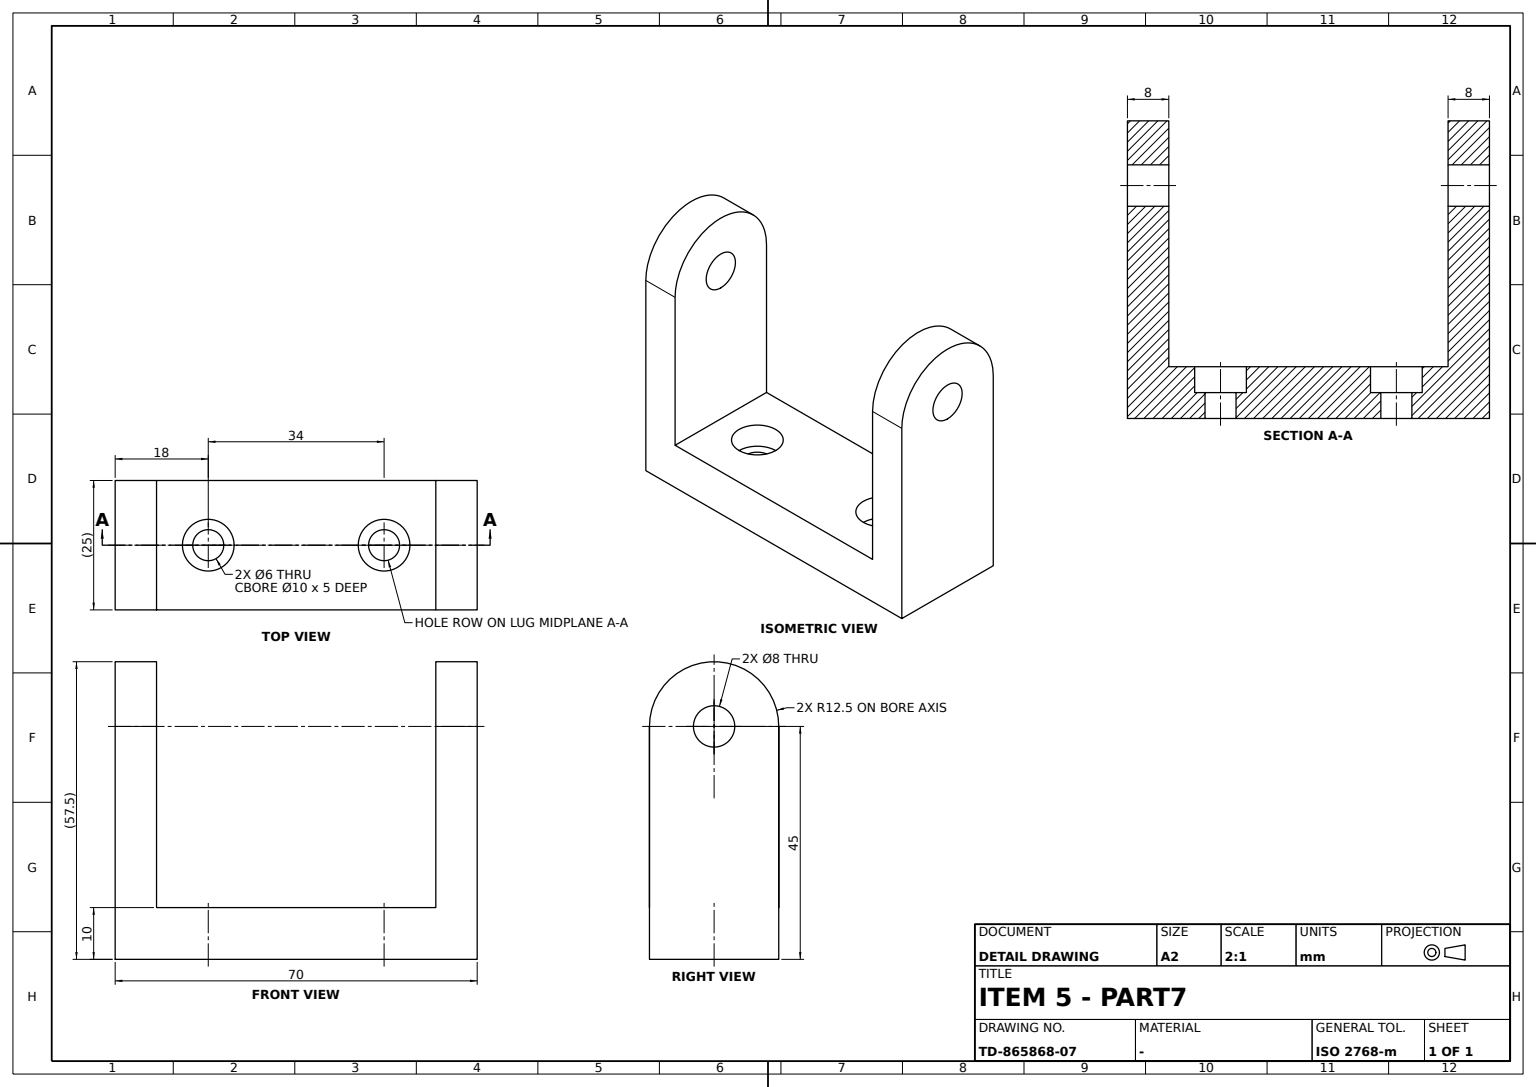
ISO-10303-21;
HEADER;
FILE_DESCRIPTION((''),'2;1');
FILE_NAME('','',(''),(''),'','','');
FILE_SCHEMA(('AUTOMOTIVE_DESIGN'));
ENDSEC;
DATA;
#1=APPLICATION_CONTEXT('');
#2=PRODUCT_CONTEXT('',#1,'mechanical');
#3=PRODUCT('','','',(#2));
#4=PRODUCT_DEFINITION_FORMATION('','',#3);
#5=PRODUCT_DEFINITION_CONTEXT('',#1,'design');
#6=PRODUCT_DEFINITION('','',#4,#5);
#7=PRODUCT_DEFINITION_SHAPE('','',#6);
#8=(LENGTH_UNIT()NAMED_UNIT(*)SI_UNIT(.MILLI.,.METRE.));
#9=(NAMED_UNIT(*)PLANE_ANGLE_UNIT()SI_UNIT($,.RADIAN.));
#10=(NAMED_UNIT(*)SI_UNIT($,.STERADIAN.)SOLID_ANGLE_UNIT());
#11=UNCERTAINTY_MEASURE_WITH_UNIT(LENGTH_MEASURE(0.005),#8,'distance_accuracy_value','');
#12=(GEOMETRIC_REPRESENTATION_CONTEXT(3)GLOBAL_UNCERTAINTY_ASSIGNED_CONTEXT((#11))GLOBAL_UNIT_ASSIGNED_CONTEXT((#8,#9,#10))REPRESENTATION_CONTEXT('',''));
#13=CARTESIAN_POINT('',(35.,0.,41.));
#14=VERTEX_POINT('',#13);
#15=CARTESIAN_POINT('',(35.,0.,45.));
#16=DIRECTION('',(1.,0.,0.));
#17=DIRECTION('',(0.,0.,-1.));
#18=AXIS2_PLACEMENT_3D('',#15,#16,#17);
#19=CIRCLE('',#18,4.);
#20=EDGE_CURVE('',#14,#14,#19,.T.);
#21=ORIENTED_EDGE('',*,*,#20,.F.);
#22=EDGE_LOOP('',(#21));
#23=FACE_BOUND('',#22,.T.);
#24=CARTESIAN_POINT('',(35.,12.5,0.));
#25=VERTEX_POINT('',#24);
#26=CARTESIAN_POINT('',(35.,12.5,45.));
#27=VERTEX_POINT('',#26);
#28=DIRECTION('',(0.,0.,1.));
#29=VECTOR('',#28,1000.);
#30=LINE('',#24,#29);
#31=EDGE_CURVE('',#25,#27,#30,.T.);
#32=ORIENTED_EDGE('',*,*,#31,.T.);
#33=CARTESIAN_POINT('',(35.,-12.5,45.));
#34=VERTEX_POINT('',#33);
#35=CIRCLE('',#18,12.5);
#36=EDGE_CURVE('',#27,#34,#35,.T.);
#37=ORIENTED_EDGE('',*,*,#36,.T.);
#38=CARTESIAN_POINT('',(35.,-12.5,0.));
#39=VERTEX_POINT('',#38);
#40=VECTOR('',#17,1000.);
#41=LINE('',#38,#40);
#42=EDGE_CURVE('',#34,#39,#41,.T.);
#43=ORIENTED_EDGE('',*,*,#42,.T.);
#44=CARTESIAN_POINT('',(35.,0.,0.));
#45=DIRECTION('',(0.,1.,0.));
#46=VECTOR('',#45,1000.);
#47=LINE('',#44,#46);
#48=EDGE_CURVE('',#39,#25,#47,.T.);
#49=ORIENTED_EDGE('',*,*,#48,.T.);
#50=EDGE_LOOP('',(#32,#37,#43,#49));
#51=FACE_BOUND('',#50,.T.);
#52=AXIS2_PLACEMENT_3D('',#44,#16,#45);
#53=PLANE('',#52);
#54=ADVANCED_FACE('',(#23,#51),#53,.T.);
#55=CARTESIAN_POINT('',(-27.,12.5,45.));
#56=VERTEX_POINT('',#55);
#57=CARTESIAN_POINT('',(-27.,-12.5,45.));
#58=VERTEX_POINT('',#57);
#59=CARTESIAN_POINT('',(-27.,0.,45.));
#60=AXIS2_PLACEMENT_3D('',#59,#16,#17);
#61=CIRCLE('',#60,12.5);
#62=EDGE_CURVE('',#56,#58,#61,.T.);
#63=ORIENTED_EDGE('',*,*,#62,.F.);
#64=CARTESIAN_POINT('',(-35.,12.5,45.));
#65=VERTEX_POINT('',#64);
#66=CARTESIAN_POINT('',(0.,12.5,45.));
#67=VECTOR('',#16,1000.);
#68=LINE('',#66,#67);
#69=EDGE_CURVE('',#65,#56,#68,.T.);
#70=ORIENTED_EDGE('',*,*,#69,.F.);
#71=CARTESIAN_POINT('',(-35.,-12.5,45.));
#72=VERTEX_POINT('',#71);
#73=CARTESIAN_POINT('',(-35.,0.,45.));
#74=AXIS2_PLACEMENT_3D('',#73,#16,#17);
#75=CIRCLE('',#74,12.5);
#76=EDGE_CURVE('',#65,#72,#75,.T.);
#77=ORIENTED_EDGE('',*,*,#76,.T.);
#78=CARTESIAN_POINT('',(0.,-12.5,45.));
#79=LINE('',#78,#67);
#80=EDGE_CURVE('',#72,#58,#79,.T.);
#81=ORIENTED_EDGE('',*,*,#80,.T.);
#82=EDGE_LOOP('',(#63,#70,#77,#81));
#83=FACE_BOUND('',#82,.T.);
#84=CARTESIAN_POINT('',(0.,0.,45.));
#85=AXIS2_PLACEMENT_3D('',#84,#16,#45);
#86=CYLINDRICAL_SURFACE('',#85,12.5);
#87=ADVANCED_FACE('',(#83),#86,.T.);
#88=CARTESIAN_POINT('',(27.,0.,49.));
#89=VERTEX_POINT('',#88);
#90=CARTESIAN_POINT('',(27.,0.,45.));
#91=DIRECTION('',(-1.,0.,0.));
#92=AXIS2_PLACEMENT_3D('',#90,#91,#28);
#93=CIRCLE('',#92,4.);
#94=EDGE_CURVE('',#89,#89,#93,.T.);
#95=ORIENTED_EDGE('',*,*,#94,.T.);
#96=EDGE_LOOP('',(#95));
#97=FACE_BOUND('',#96,.T.);
#98=ORIENTED_EDGE('',*,*,#20,.T.);
#99=EDGE_LOOP('',(#98));
#100=FACE_BOUND('',#99,.T.);
#101=CYLINDRICAL_SURFACE('',#85,4.);
#102=ADVANCED_FACE('',(#97,#100),#101,.F.);
#103=CARTESIAN_POINT('',(-27.,12.5,10.));
#104=VERTEX_POINT('',#103);
#105=LINE('',#103,#29);
#106=EDGE_CURVE('',#104,#56,#105,.T.);
#107=ORIENTED_EDGE('',*,*,#106,.F.);
#108=CARTESIAN_POINT('',(27.,12.5,10.));
#109=VERTEX_POINT('',#108);
#110=LINE('',#103,#67);
#111=EDGE_CURVE('',#104,#109,#110,.T.);
#112=ORIENTED_EDGE('',*,*,#111,.T.);
#113=CARTESIAN_POINT('',(27.,12.5,45.));
#114=VERTEX_POINT('',#113);
#115=CARTESIAN_POINT('',(27.,12.5,63.142235));
#116=LINE('',#115,#40);
#117=EDGE_CURVE('',#114,#109,#116,.T.);
#118=ORIENTED_EDGE('',*,*,#117,.F.);
#119=EDGE_CURVE('',#114,#27,#68,.T.);
#120=ORIENTED_EDGE('',*,*,#119,.T.);
#121=ORIENTED_EDGE('',*,*,#31,.F.);
#122=CARTESIAN_POINT('',(-35.,12.5,0.));
#123=VERTEX_POINT('',#122);
#124=CARTESIAN_POINT('',(0.,12.5,0.));
#125=LINE('',#124,#67);
#126=EDGE_CURVE('',#123,#25,#125,.T.);
#127=ORIENTED_EDGE('',*,*,#126,.F.);
#128=LINE('',#122,#29);
#129=EDGE_CURVE('',#123,#65,#128,.T.);
#130=ORIENTED_EDGE('',*,*,#129,.T.);
#131=ORIENTED_EDGE('',*,*,#69,.T.);
#132=EDGE_LOOP('',(#107,#112,#118,#120,#121,#127,#130,#131));
#133=FACE_BOUND('',#132,.T.);
#134=AXIS2_PLACEMENT_3D('',#124,#45,#28);
#135=PLANE('',#134);
#136=ADVANCED_FACE('',(#133),#135,.T.);
#137=CARTESIAN_POINT('',(-35.,-12.5,0.));
#138=VERTEX_POINT('',#137);
#139=LINE('',#137,#40);
#140=EDGE_CURVE('',#72,#138,#139,.T.);
#141=ORIENTED_EDGE('',*,*,#140,.F.);
#142=ORIENTED_EDGE('',*,*,#76,.F.);
#143=ORIENTED_EDGE('',*,*,#129,.F.);
#144=CARTESIAN_POINT('',(-35.,0.,0.));
#145=LINE('',#144,#46);
#146=EDGE_CURVE('',#138,#123,#145,.T.);
#147=ORIENTED_EDGE('',*,*,#146,.F.);
#148=EDGE_LOOP('',(#141,#142,#143,#147));
#149=FACE_BOUND('',#148,.T.);
#150=CARTESIAN_POINT('',(-35.,0.,41.));
#151=VERTEX_POINT('',#150);
#152=CIRCLE('',#74,4.);
#153=EDGE_CURVE('',#151,#151,#152,.T.);
#154=ORIENTED_EDGE('',*,*,#153,.T.);
#155=EDGE_LOOP('',(#154));
#156=FACE_BOUND('',#155,.T.);
#157=AXIS2_PLACEMENT_3D('',#144,#16,#45);
#158=PLANE('',#157);
#159=ADVANCED_FACE('',(#149,#156),#158,.F.);
#160=CARTESIAN_POINT('',(-14.,0.,5.));
#161=VERTEX_POINT('',#160);
#162=CARTESIAN_POINT('',(-17.,0.,5.));
#163=AXIS2_PLACEMENT_3D('',#162,#28,#16);
#164=CIRCLE('',#163,3.);
#165=EDGE_CURVE('',#161,#161,#164,.T.);
#166=ORIENTED_EDGE('',*,*,#165,.T.);
#167=EDGE_LOOP('',(#166));
#168=FACE_BOUND('',#167,.T.);
#169=CARTESIAN_POINT('',(-20.,0.,0.));
#170=VERTEX_POINT('',#169);
#171=CARTESIAN_POINT('',(-17.,0.,0.));
#172=AXIS2_PLACEMENT_3D('',#171,#17,#91);
#173=CIRCLE('',#172,3.);
#174=EDGE_CURVE('',#170,#170,#173,.F.);
#175=ORIENTED_EDGE('',*,*,#174,.F.);
#176=EDGE_LOOP('',(#175));
#177=FACE_BOUND('',#176,.T.);
#178=CARTESIAN_POINT('',(-17.,0.,2.5));
#179=AXIS2_PLACEMENT_3D('',#178,#28,#16);
#180=CYLINDRICAL_SURFACE('',#179,3.);
#181=ADVANCED_FACE('',(#168,#177),#180,.F.);
#182=CARTESIAN_POINT('',(12.,0.,10.));
#183=VERTEX_POINT('',#182);
#184=CARTESIAN_POINT('',(17.,0.,10.));
#185=AXIS2_PLACEMENT_3D('',#184,#17,#91);
#186=CIRCLE('',#185,5.);
#187=EDGE_CURVE('',#183,#183,#186,.F.);
#188=ORIENTED_EDGE('',*,*,#187,.T.);
#189=EDGE_LOOP('',(#188));
#190=FACE_BOUND('',#189,.T.);
#191=CARTESIAN_POINT('',(22.,0.,5.));
#192=VERTEX_POINT('',#191);
#193=CARTESIAN_POINT('',(17.,0.,5.));
#194=AXIS2_PLACEMENT_3D('',#193,#28,#16);
#195=CIRCLE('',#194,5.);
#196=EDGE_CURVE('',#192,#192,#195,.T.);
#197=ORIENTED_EDGE('',*,*,#196,.F.);
#198=EDGE_LOOP('',(#197));
#199=FACE_BOUND('',#198,.T.);
#200=CARTESIAN_POINT('',(17.,0.,7.5));
#201=AXIS2_PLACEMENT_3D('',#200,#28,#16);
#202=CYLINDRICAL_SURFACE('',#201,5.);
#203=ADVANCED_FACE('',(#190,#199),#202,.F.);
#204=CARTESIAN_POINT('',(-22.,0.,10.));
#205=VERTEX_POINT('',#204);
#206=CARTESIAN_POINT('',(-17.,0.,10.));
#207=AXIS2_PLACEMENT_3D('',#206,#17,#91);
#208=CIRCLE('',#207,5.);
#209=EDGE_CURVE('',#205,#205,#208,.F.);
#210=ORIENTED_EDGE('',*,*,#209,.T.);
#211=EDGE_LOOP('',(#210));
#212=FACE_BOUND('',#211,.T.);
#213=CARTESIAN_POINT('',(-12.,0.,5.));
#214=VERTEX_POINT('',#213);
#215=CIRCLE('',#163,5.);
#216=EDGE_CURVE('',#214,#214,#215,.T.);
#217=ORIENTED_EDGE('',*,*,#216,.F.);
#218=EDGE_LOOP('',(#217));
#219=FACE_BOUND('',#218,.T.);
#220=CARTESIAN_POINT('',(-17.,0.,7.5));
#221=AXIS2_PLACEMENT_3D('',#220,#28,#16);
#222=CYLINDRICAL_SURFACE('',#221,5.);
#223=ADVANCED_FACE('',(#212,#219),#222,.F.);
#224=ORIENTED_EDGE('',*,*,#119,.F.);
#225=CARTESIAN_POINT('',(27.,-12.5,45.));
#226=VERTEX_POINT('',#225);
#227=CIRCLE('',#92,12.5);
#228=EDGE_CURVE('',#226,#114,#227,.T.);
#229=ORIENTED_EDGE('',*,*,#228,.F.);
#230=EDGE_CURVE('',#226,#34,#79,.T.);
#231=ORIENTED_EDGE('',*,*,#230,.T.);
#232=ORIENTED_EDGE('',*,*,#36,.F.);
#233=EDGE_LOOP('',(#224,#229,#231,#232));
#234=FACE_BOUND('',#233,.T.);
#235=ADVANCED_FACE('',(#234),#86,.T.);
#236=CARTESIAN_POINT('',(-27.,-12.5,10.));
#237=VERTEX_POINT('',#236);
#238=CARTESIAN_POINT('',(27.,-12.5,10.));
#239=VERTEX_POINT('',#238);
#240=CARTESIAN_POINT('',(0.,-12.5,10.));
#241=LINE('',#240,#67);
#242=EDGE_CURVE('',#237,#239,#241,.T.);
#243=ORIENTED_EDGE('',*,*,#242,.F.);
#244=LINE('',#236,#40);
#245=EDGE_CURVE('',#58,#237,#244,.T.);
#246=ORIENTED_EDGE('',*,*,#245,.F.);
#247=ORIENTED_EDGE('',*,*,#80,.F.);
#248=ORIENTED_EDGE('',*,*,#140,.T.);
#249=CARTESIAN_POINT('',(0.,-12.5,0.));
#250=LINE('',#249,#67);
#251=EDGE_CURVE('',#138,#39,#250,.T.);
#252=ORIENTED_EDGE('',*,*,#251,.T.);
#253=ORIENTED_EDGE('',*,*,#42,.F.);
#254=ORIENTED_EDGE('',*,*,#230,.F.);
#255=LINE('',#225,#40);
#256=EDGE_CURVE('',#226,#239,#255,.T.);
#257=ORIENTED_EDGE('',*,*,#256,.T.);
#258=EDGE_LOOP('',(#243,#246,#247,#248,#252,#253,#254,#257));
#259=FACE_BOUND('',#258,.T.);
#260=DIRECTION('',(0.,-1.,0.));
#261=AXIS2_PLACEMENT_3D('',#78,#260,#17);
#262=PLANE('',#261);
#263=ADVANCED_FACE('',(#259),#262,.T.);
#264=CARTESIAN_POINT('',(14.,0.,0.));
#265=VERTEX_POINT('',#264);
#266=CARTESIAN_POINT('',(17.,0.,0.));
#267=AXIS2_PLACEMENT_3D('',#266,#17,#91);
#268=CIRCLE('',#267,3.);
#269=EDGE_CURVE('',#265,#265,#268,.F.);
#270=ORIENTED_EDGE('',*,*,#269,.T.);
#271=EDGE_LOOP('',(#270));
#272=FACE_BOUND('',#271,.T.);
#273=ORIENTED_EDGE('',*,*,#174,.T.);
#274=EDGE_LOOP('',(#273));
#275=FACE_BOUND('',#274,.T.);
#276=ORIENTED_EDGE('',*,*,#48,.F.);
#277=ORIENTED_EDGE('',*,*,#251,.F.);
#278=ORIENTED_EDGE('',*,*,#146,.T.);
#279=ORIENTED_EDGE('',*,*,#126,.T.);
#280=EDGE_LOOP('',(#276,#277,#278,#279));
#281=FACE_BOUND('',#280,.T.);
#282=AXIS2_PLACEMENT_3D('',#249,#17,#45);
#283=PLANE('',#282);
#284=ADVANCED_FACE('',(#272,#275,#281),#283,.T.);
#285=ORIENTED_EDGE('',*,*,#165,.F.);
#286=EDGE_LOOP('',(#285));
#287=FACE_BOUND('',#286,.T.);
#288=ORIENTED_EDGE('',*,*,#216,.T.);
#289=EDGE_LOOP('',(#288));
#290=FACE_BOUND('',#289,.T.);
#291=CARTESIAN_POINT('',(0.,0.,5.));
#292=AXIS2_PLACEMENT_3D('',#291,#28,#16);
#293=PLANE('',#292);
#294=ADVANCED_FACE('',(#287,#290),#293,.T.);
#295=ORIENTED_EDGE('',*,*,#94,.F.);
#296=EDGE_LOOP('',(#295));
#297=FACE_BOUND('',#296,.T.);
#298=ORIENTED_EDGE('',*,*,#228,.T.);
#299=ORIENTED_EDGE('',*,*,#117,.T.);
#300=VECTOR('',#260,1000.);
#301=LINE('',#108,#300);
#302=EDGE_CURVE('',#109,#239,#301,.T.);
#303=ORIENTED_EDGE('',*,*,#302,.T.);
#304=ORIENTED_EDGE('',*,*,#256,.F.);
#305=EDGE_LOOP('',(#298,#299,#303,#304));
#306=FACE_BOUND('',#305,.T.);
#307=AXIS2_PLACEMENT_3D('',#115,#91,#17);
#308=PLANE('',#307);
#309=ADVANCED_FACE('',(#297,#306),#308,.T.);
#310=ORIENTED_EDGE('',*,*,#187,.F.);
#311=EDGE_LOOP('',(#310));
#312=FACE_BOUND('',#311,.T.);
#313=ORIENTED_EDGE('',*,*,#209,.F.);
#314=EDGE_LOOP('',(#313));
#315=FACE_BOUND('',#314,.T.);
#316=ORIENTED_EDGE('',*,*,#111,.F.);
#317=LINE('',#103,#300);
#318=EDGE_CURVE('',#104,#237,#317,.T.);
#319=ORIENTED_EDGE('',*,*,#318,.T.);
#320=ORIENTED_EDGE('',*,*,#242,.T.);
#321=ORIENTED_EDGE('',*,*,#302,.F.);
#322=EDGE_LOOP('',(#316,#319,#320,#321));
#323=FACE_BOUND('',#322,.T.);
#324=AXIS2_PLACEMENT_3D('',#103,#17,#16);
#325=PLANE('',#324);
#326=ADVANCED_FACE('',(#312,#315,#323),#325,.F.);
#327=ORIENTED_EDGE('',*,*,#153,.F.);
#328=EDGE_LOOP('',(#327));
#329=FACE_BOUND('',#328,.T.);
#330=CARTESIAN_POINT('',(-27.,0.,41.));
#331=VERTEX_POINT('',#330);
#332=CIRCLE('',#60,4.);
#333=EDGE_CURVE('',#331,#331,#332,.T.);
#334=ORIENTED_EDGE('',*,*,#333,.T.);
#335=EDGE_LOOP('',(#334));
#336=FACE_BOUND('',#335,.T.);
#337=ADVANCED_FACE('',(#329,#336),#101,.F.);
#338=ORIENTED_EDGE('',*,*,#196,.T.);
#339=EDGE_LOOP('',(#338));
#340=FACE_BOUND('',#339,.T.);
#341=CARTESIAN_POINT('',(20.,0.,5.));
#342=VERTEX_POINT('',#341);
#343=CIRCLE('',#194,3.);
#344=EDGE_CURVE('',#342,#342,#343,.T.);
#345=ORIENTED_EDGE('',*,*,#344,.F.);
#346=EDGE_LOOP('',(#345));
#347=FACE_BOUND('',#346,.T.);
#348=ADVANCED_FACE('',(#340,#347),#293,.T.);
#349=ORIENTED_EDGE('',*,*,#269,.F.);
#350=EDGE_LOOP('',(#349));
#351=FACE_BOUND('',#350,.T.);
#352=ORIENTED_EDGE('',*,*,#344,.T.);
#353=EDGE_LOOP('',(#352));
#354=FACE_BOUND('',#353,.T.);
#355=CARTESIAN_POINT('',(17.,0.,2.5));
#356=AXIS2_PLACEMENT_3D('',#355,#28,#16);
#357=CYLINDRICAL_SURFACE('',#356,3.);
#358=ADVANCED_FACE('',(#351,#354),#357,.F.);
#359=ORIENTED_EDGE('',*,*,#333,.F.);
#360=EDGE_LOOP('',(#359));
#361=FACE_BOUND('',#360,.T.);
#362=ORIENTED_EDGE('',*,*,#106,.T.);
#363=ORIENTED_EDGE('',*,*,#62,.T.);
#364=ORIENTED_EDGE('',*,*,#245,.T.);
#365=ORIENTED_EDGE('',*,*,#318,.F.);
#366=EDGE_LOOP('',(#362,#363,#364,#365));
#367=FACE_BOUND('',#366,.T.);
#368=AXIS2_PLACEMENT_3D('',#103,#16,#28);
#369=PLANE('',#368);
#370=ADVANCED_FACE('',(#361,#367),#369,.T.);
#371=CLOSED_SHELL('',(#54,#87,#102,#136,#159,#181,#203,#223,#235,#263,#284,#294,#309,#326,#337,#348,#358,#370));
#372=MANIFOLD_SOLID_BREP('',#371);
#373=ADVANCED_BREP_SHAPE_REPRESENTATION('',(#372),#12);
#374=SHAPE_DEFINITION_REPRESENTATION(#7,#373);
ENDSEC;
END-ISO-10303-21;
